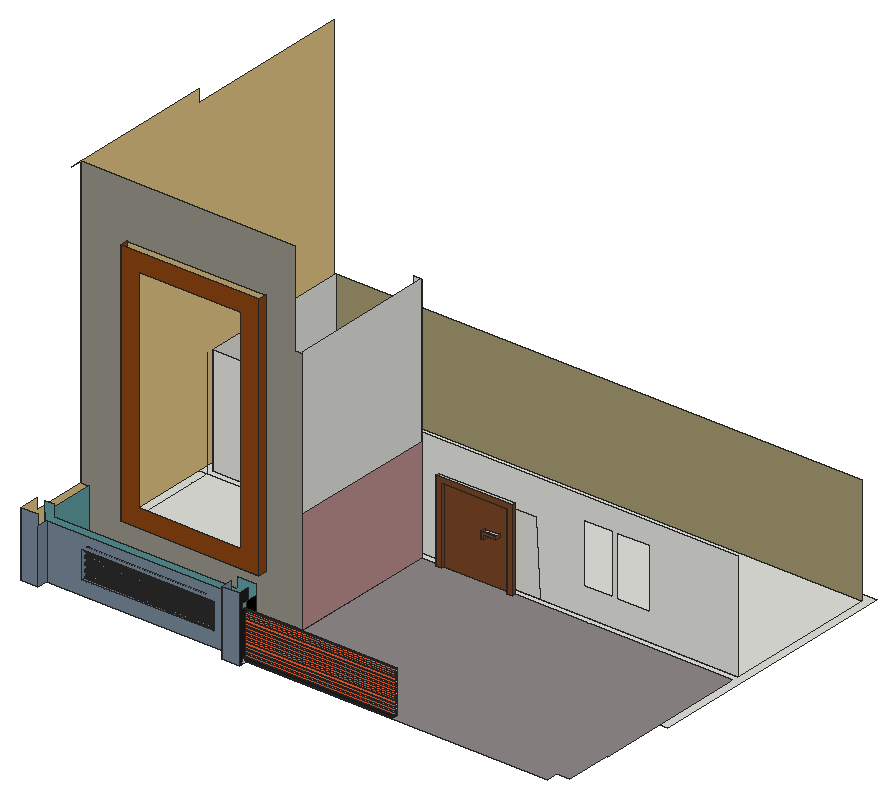
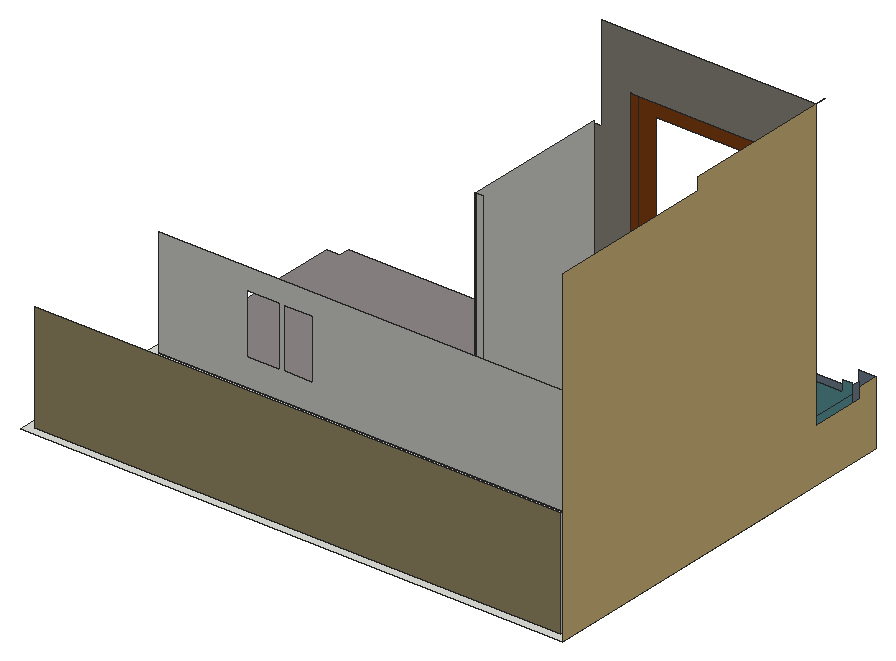
# SketchUp Ruby script. Lengths in inches.
U = 1.inch
M = Sketchup.active_model
def pt(a) = Geom::Point3d.new(a.map { |v| v * U })
def face(e, loops, mat)
  f = e.add_face(loops[0].map { |a| pt(a) })
  loops[1..].each { |l| e.add_face(l.map { |a| pt(a) }).erase! }
  f.material = f.back_material = mat if mat
  f
end
# faces: each face lists its corners as indices into pts; further lists are holes
def faces(e, pts, list, mat = nil) = list.each { |f| face(e, (f[0].is_a?(Array) ? f : [f]).map { |l| l.map { |i| pts[i] } }, mat) }
# xy, xz, yz: faces in a plane at the given z, y or x. An outline is a flat list of corners, or four numbers for a rectangle; further outlines are holes
def ring(l) = l.size == 4 ? [[l[0], l[1]], [l[2], l[1]], [l[2], l[3]], [l[0], l[3]]] : l.each_slice(2).to_a
def flat(e, list, mat, &to3) = list.each { |f| face(e, (f[0].is_a?(Array) ? f : [f]).map { |l| ring(l).map { |u, v| to3.(u, v) } }, mat) }
def xy(e, z, list, mat = nil) = flat(e, list, mat) { |x, y| [x, y, z] }
def xz(e, y, list, mat = nil) = flat(e, list, mat) { |x, z| [x, y, z] }
def yz(e, x, list, mat = nil) = flat(e, list, mat) { |y, z| [x, y, z] }
def lines(e, pts, list) = list.each { |a, b| e.add_line(pt(pts[a]), pt(pts[b])) }
# prism: a flat outline (further loops are holes) pulled along v
def prism(e, loops, v, mat = nil)
  f = face(e, loops, mat); d = Geom::Vector3d.new(v.map { |x| x * U })
  f.pushpull(f.normal.samedirection?(d) ? d.length : -d.length)
end
def box(e, o, s, mat = nil) = prism(e, [[o, [o[0] + s[0], o[1], o[2]], [o[0] + s[0], o[1] + s[1], o[2]], [o[0], o[1] + s[1], o[2]]]], [0, 0, s[2]], mat)
def at(x, y, z, deg = 0) = Geom::Transformation.translation(pt([x, y, z])) * Geom::Transformation.rotation(ORIGIN, Z_AXIS, deg.degrees)
def axes(o, x, y, z) = Geom::Transformation.new([*x, 0, *y, 0, *z, 0, *pt(o).to_a, 1])
def part(name) = M.definitions.add(name)
# library, detail: a bought-in or finely detailed component or shape, given as its bounding box
def library(name, o, s) = part(name).tap { |d| box(d.entities, o, s) }
def detail(e, o, s) = box(e.add_group.entities, o, s)
def put(e, d, t, mat = nil) = e.add_instance(d, t).tap { |i| i.material = mat if mat }
def group(e, t, mat = nil) = e.add_group.tap { |g| g.transformation = t; g.material = mat if mat }.entities
root = M.entities
M.materials.add("[0043_SaddleBrown]").color = [139, 69, 19]
M.materials.add("[0081_CadetBlue]").color = [95, 158, 160]
M.materials.add("[0110_LightSlateGray]").color = [119, 136, 153]
M.materials.add("[0119_RosyBrown]").color = [188, 143, 143]
M.materials.add("[0137_Black]").color = [0, 0, 0]
M.materials.add("[Color B04]").color = [255, 101, 50]
M.materials.add("[Color M08]").color = [30, 30, 30]
M.materials.add("[Concrete Aggregate Smoke]").color = [154, 150, 148]
M.materials.add("[Formica Graystone]").color = [149, 146, 135]
M.materials.add("[Stone Brushed Khaki]").color = [226, 197, 133]
M.materials.add("[Stone Marble]").color = [143, 138, 136]
M.materials.add("[Wood Lumber ButtJoined]").color = [164, 152, 112]
M.materials.add("[Wood Veneer 01]").color = [120, 70, 37]
xy(root,-0.6875,[[249.488,83.423,257.613,247.17]])
xy(root,0,[[12,0,12,83.423,21.531,83.423,21.531,22.384,254.581,22.384,254.581,0,235.107,0,235.107,12,31.287,12,31.287,0],[12,83.423,21,135.461],[21,83.423,249.488,135.461],[249.488,83.423,257.613,135.461],[257.613,83.423,258.19,135.461],
  [12,135.461,21,145.845],[21,135.461,249.488,145.845],[249.488,135.461,257.613,145.845],[257.613,135.461,258.19,145.845],[12,145.845,21,247.17],
  [[603,145.845,603,247.17,355.224,247.17,355.224,250.17,283.224,250.17,283.224,247.17,12,247.17,12,434.423,612,434.423,612,145.845],[21,254.423,603,425.423]],[21,145.845,249.488,247.17],[249.488,145.845,257.613,247.17],[257.613,145.845,258.19,247.17],[276.992,244.17,283.224,247.17],
  [355.224,244.17,361.455,247.17],[283.224,247.17,355.224,250.17],[21,254.423,603,425.423]])
xy(root,0,[[254.581,9.884,587.783,9.884,587.783,22.384,602.489,22.384,602.489,74.423,603,74.423,603,247.17,361.455,247.17,361.455,244.17,355.224,244.17,355.224,247.17,283.224,247.17,283.224,244.17,276.992,244.17,276.992,247.17,258.19,247.17,258.19,83.423,21.531,83.423,21.531,22.384,254.581,22.384]],"[Stone Marble]")
xy(root,4.99,[[254.581,3.884,421.182,9.884]],"[Color M08]")
xy(root,6.884,[[254.581,6.884,420.872,9.884]],"[Color B04]")
xy(root,8.996,[[254.581,6.884,420.872,9.884]],"[Color B04]")
xy(root,10.576,[[254.581,6.884,421.182,9.884]],"[Color B04]")
xy(root,12.688,[[254.581,6.884,421.182,9.884]],"[Color B04]")
xy(root,14.451,[[254.581,6.884,421.182,9.884]],"[Color B04]")
xy(root,15.741,[[70.247,15.6,216.31,19.453],[216.31,15.6,221.935,19.453],[70.247,19.453,216.31,22.384]])
xy(root,15.741,[[70.247,12,216.31,15.6]],"[0110_LightSlateGray]")
xy(root,16.563,[[254.581,6.884,421.182,9.884]],"[Color B04]")
xy(root,18.263,[[254.581,6.884,421.182,9.884]],"[Color B04]")
xy(root,20.375,[[254.581,6.884,421.182,9.884]],"[Color B04]")
xy(root,22.076,[[254.581,6.884,421.182,9.884]],"[Color B04]")
xy(root,24.188,[[254.581,6.884,421.182,9.884]],"[Color B04]")
xy(root,25.888,[[254.581,6.884,421.182,9.884]],"[Color B04]")
xy(root,28,[[254.581,6.884,421.182,9.884]],"[Color B04]")
xy(root,29.701,[[254.581,6.884,421.182,9.884]],"[Color B04]")
xy(root,31.813,[[254.581,6.884,421.182,9.884]],"[Color B04]")
xy(root,33.513,[[254.581,6.884,421.182,9.884]],"[Color B04]")
xy(root,35.625,[[254.581,6.884,421.182,9.884]],"[Color B04]")
xy(root,37.326,[[254.581,6.884,421.182,9.884]],"[Color B04]")
xy(root,39.438,[[254.581,6.884,421.182,9.884]],"[Color B04]")
xy(root,41.138,[[254.581,6.884,421.182,9.884]],"[Color B04]")
xy(root,43.25,[[254.581,6.884,421.182,9.884]],"[Color B04]")
xy(root,43.565,[[63.349,74.423,216.911,83.423]])
xy(root,44.951,[[254.581,6.884,421.182,9.884]],"[Color B04]")
xy(root,45.804,[[70.247,12,216.31,22.384]],"[0110_LightSlateGray]")
xy(root,46.461,[[328.975,241.17,331.645,247.17]],"[Wood Veneer 01]")
xy(root,47.063,[[254.581,6.884,421.182,9.884]],"[Color B04]")
xy(root,48.763,[[254.581,6.884,421.182,9.884]],"[Color B04]")
xy(root,50.875,[[254.581,6.884,421.182,9.884]],"[Color B04]")
xy(root,50.899,[[331.645,241.17,345.538,247.17]],"[Wood Veneer 01]")
xz(root,0,[[12,0,31.287,0,31.287,60,31.228,60,31.228,72,12,72],[235.107,0,254.581,72]],"[0110_LightSlateGray]")
xz(root,6.884,[[254.581,6.884,420.872,8.996],[254.581,10.576,421.182,12.688],[254.581,14.451,421.182,16.563],[254.581,18.263,421.182,20.375],[254.581,22.076,421.182,24.188],
  [254.581,25.888,421.182,28],[254.581,29.701,421.182,31.813],[254.581,33.513,421.182,35.625],[254.581,37.326,421.182,39.438],[254.581,41.138,421.182,43.25],
  [254.581,44.951,421.182,47.063],[254.581,48.763,421.182,50.875]],"[Color B04]")
xz(root,9.884,[[251.209,6.884,254.581,8.996],[254.581,6.884,417.81,8.996],[254.581,10.576,421.182,12.688],[254.581,14.451,421.182,16.563],[254.581,18.263,421.182,20.375],
  [254.581,22.076,421.182,24.188],[254.581,25.888,421.182,28],[254.581,29.701,421.182,31.813],[254.581,33.513,421.182,35.625],[254.581,37.326,421.182,39.438],
  [254.581,41.138,421.182,43.25],[254.581,44.951,421.182,47.063],[254.581,48.763,421.182,50.875]])
xz(root,9.884,[[254.581,4.99,421.182,4.99,421.182,10.576,254.581,10.576,254.581,8.996,420.872,8.996,420.872,6.884,254.581,6.884],[254.581,12.688,421.182,14.451],[254.581,16.563,421.182,18.263],[254.581,20.375,421.182,22.076],[254.581,24.188,421.182,25.888],
  [254.581,28,421.182,29.701],[254.581,31.813,421.182,33.513],[254.581,35.625,421.182,37.326],[254.581,39.438,421.182,41.138],[254.581,43.25,421.182,44.951],
  [254.581,47.063,421.182,48.763],[254.581,50.875,421.182,52.576]],"[Color B04]")
xz(root,12,[[[31.287,0,235.107,60],[70.247,15.741,216.31,45.804]]],"[0110_LightSlateGray]")
xz(root,22.384,[[[21.531,0,21.531,72,31.228,72,31.228,60,235.107,60,235.107,72,254.584,72,254.584,60,254.581,60,254.581,0],[70.247,15.741,216.31,45.804]]],"[0081_CadetBlue]")
xz(root,74.423,[[[63.349,43.565,216.911,317.69],[83.364,63.579,196.897,297.675]]],"[0043_SaddleBrown]")
xz(root,83.423,[[249.488,-0.6875,257.613,0],[21,0,21.531,60],[257.613,0,258.19,273.75]])
xz(root,83.423,[[[21.531,0,257.613,0,257.613,273.75,249.488,273.75,249.488,378.517,12,378.517,12,60,21.531,60],[63.349,43.565,216.911,317.69]]],"[Formica Graystone]")
xz(root,241.17,[[328.975,46.461,331.645,46.461,331.645,50.899,345.538,50.899,345.538,53.899,328.975,53.899]],"[Wood Veneer 01]")
xz(root,244.17,[[276.992,0,283.224,0,283.224,84,355.224,84,355.224,0,361.455,0,361.455,90.231,276.992,90.231]],"[Wood Veneer 01]")
xz(root,247.17,[[249.488,-0.6875,257.613,0],[249.488,0,257.613,276],[257.613,0,258.19,276],[276.992,0,276.992,90.231,361.455,90.231,361.455,0,355.224,0,355.224,84,283.224,84,283.224,0],[328.975,46.461,328.975,53.899,345.538,53.899,345.538,50.899,331.645,50.899,331.645,46.461]])
xz(root,247.17,[[[283.224,0,355.224,84],[328.975,46.461,328.975,53.899,345.538,53.899,345.538,50.899,331.645,50.899,331.645,46.461]]],"[Wood Veneer 01]")
xz(root,250.17,[[283.224,0,355.224,84]])
xz(root,254.423,[[[21,0,603,120],[468.879,30.198,505.379,95.948],[432.379,30.198,464.497,95.948]]])
xz(root,425.423,[[21,0,603,120]],"[Wood Lumber ButtJoined]")
yz(root,12,[[0,0,0,72,22.384,72,22.384,60,83.423,60,83.423,378.517,71.423,378.517,71.423,378.735,247.17,378.735,247.17,364.4375,434.423,364.4375,434.423,0]],"[Stone Brushed Khaki]")
yz(root,21,[[254.423,0,425.423,120]])
yz(root,21.531,[[22.384,0,83.423,60]],"[0081_CadetBlue]")
yz(root,31.287,[[0,0,12,60]],"[0110_LightSlateGray]")
yz(root,63.349,[[74.423,43.565,83.423,317.69]],"[0043_SaddleBrown]")
yz(root,70.247,[[17.526,14.371,18.06,14.441,18.558,14.647,18.985,14.975,19.3125,15.402,19.453,15.741,15.6,15.741,15.74,15.402,16.068,14.975,16.495,14.647,16.992,14.441]])
yz(root,70.247,[[[12,15.741,15.6,15.741,15.534,15.899,15.464,16.433,15.534,16.967,15.74,17.465,16.068,17.892,16.495,18.219,16.992,18.425,17.526,18.496,18.06,18.425,18.558,18.219,18.985,17.892,19.3125,17.465,19.518,16.967,19.589,16.433,19.518,15.899,19.453,15.741,22.384,15.741,22.384,45.804,12,45.804],[17.526,41.121,16.992,41.191,16.495,41.397,16.068,41.725,15.74,42.152,15.534,42.649,15.464,43.183,15.534,43.717,15.74,44.215,16.068,44.642,16.495,44.969,16.992,45.175,17.526,45.246,18.06,45.175,18.558,44.969,18.985,44.642,19.3125,44.215,19.518,43.717,19.589,43.183,19.518,42.649,19.3125,42.152,18.985,41.725,18.558,41.397,18.06,41.191],[17.526,34.433,16.992,34.504,16.495,34.71,16.068,35.037,15.74,35.465,15.534,35.962,15.464,36.496,15.534,37.03,15.74,37.527,16.068,37.954,16.495,38.282,16.992,38.488,17.526,38.558,18.06,38.488,18.558,38.282,18.985,37.954,19.3125,37.527,19.518,37.03,19.589,36.496,19.518,35.962,19.3125,35.465,18.985,35.037,18.558,34.71,18.06,34.504],[17.526,27.746,16.992,27.816,16.495,28.022,16.068,28.35,15.74,28.777,15.534,29.274,15.464,29.808,15.534,30.342,15.74,30.84,16.068,31.267,16.495,31.594,16.992,31.8,17.526,31.871,18.06,31.8,18.558,31.594,18.985,31.267,19.3125,30.84,19.518,30.342,19.589,29.808,19.518,29.274,19.3125,28.777,18.985,28.35,18.558,28.022,18.06,27.816],[17.526,21.058,16.992,21.129,16.495,21.335,16.068,21.662,15.74,22.09,15.534,22.587,15.464,23.121,15.534,23.655,15.74,24.152,16.068,24.579,16.495,24.907,16.992,25.113,17.526,25.183,18.06,25.113,18.558,24.907,18.985,24.579,19.3125,24.152,19.518,23.655,19.589,23.121,19.518,22.587,19.3125,22.09,18.985,21.662,18.558,21.335,18.06,21.129]]],"[0110_LightSlateGray]")
yz(root,216.31,[[[12,15.741,22.384,45.804],[17.526,27.746,18.06,27.816,18.558,28.022,18.985,28.35,19.3125,28.777,19.518,29.274,19.589,29.808,19.518,30.342,19.3125,30.84,18.985,31.267,18.558,31.594,18.06,31.8,17.526,31.871,16.992,31.8,16.495,31.594,16.068,31.267,15.74,30.84,15.534,30.342,15.464,29.808,15.534,29.274,15.74,28.777,16.068,28.35,16.495,28.022,16.992,27.816]]],"[0110_LightSlateGray]")
yz(root,216.911,[[74.423,43.565,83.423,317.69]],"[0043_SaddleBrown]")
yz(root,218.997,[[17.526,21.058,18.06,21.129,18.558,21.335,18.985,21.662,19.3125,22.09,19.518,22.587,19.589,23.121,19.518,23.655,19.3125,24.152,18.985,24.579,18.558,24.907,18.06,25.113,17.526,25.183,16.992,25.113,16.495,24.907,16.068,24.579,15.74,24.152,15.534,23.655,15.464,23.121,15.534,22.587,15.74,22.09,16.068,21.662,16.495,21.335,16.992,21.129]])
yz(root,220.497,[[17.526,41.121,18.06,41.191,18.558,41.397,18.985,41.725,19.3125,42.152,19.518,42.649,19.589,43.183,19.518,43.717,19.3125,44.215,18.985,44.642,18.558,44.969,18.06,45.175,17.526,45.246,16.992,45.175,16.495,44.969,16.068,44.642,15.74,44.215,15.534,43.717,15.464,43.183,15.534,42.649,15.74,42.152,16.068,41.725,16.495,41.397,16.992,41.191]])
yz(root,221.935,[[15.6,15.741,19.453,15.741,19.518,15.899,19.589,16.433,19.518,16.967,19.3125,17.465,18.985,17.892,18.558,18.219,18.06,18.425,17.526,18.496,16.992,18.425,16.495,18.219,16.068,17.892,15.74,17.465,15.534,16.967,15.464,16.433,15.534,15.899]])
yz(root,223.872,[[17.526,34.433,18.06,34.504,18.558,34.71,18.985,35.037,19.3125,35.465,19.518,35.962,19.589,36.496,19.518,37.03,19.3125,37.527,18.985,37.954,18.558,38.282,18.06,38.488,17.526,38.558,16.992,38.488,16.495,38.282,16.068,37.954,15.74,37.527,15.534,37.03,15.464,36.496,15.534,35.962,15.74,35.465,16.068,35.037,16.495,34.71,16.992,34.504]])
yz(root,235.107,[[0,0,12,72]],"[0110_LightSlateGray]")
yz(root,249.488,[[83.423,-0.6875,247.17,0]])
yz(root,254.581,[[3.884,0,6.884,4.99],[6.884,0,9.884,4.99],[6.884,6.884,9.884,8.996],[6.884,10.576,9.884,12.688],[6.884,14.451,9.884,16.563],
  [6.884,18.263,9.884,20.375],[6.884,22.076,9.884,24.188],[6.884,25.888,9.884,28],[6.884,29.701,9.884,31.813],[6.884,33.513,9.884,35.625],
  [6.884,37.326,9.884,39.438],[6.884,41.138,9.884,43.25],[6.884,44.951,9.884,47.063],[6.884,48.763,9.884,50.875]])
yz(root,254.581,[[9.884,0,22.384,60]],"[0137_Black]")
yz(root,254.581,[[0,0,3.884,0,3.884,4.99,9.884,4.99,9.884,6.884,6.884,6.884,6.884,8.996,9.884,8.996,9.884,10.576,6.884,10.576,6.884,12.688,9.884,12.688,9.884,14.451,6.884,14.451,6.884,16.563,9.884,16.563,9.884,18.263,6.884,18.263,6.884,20.375,9.884,20.375,9.884,22.076,6.884,22.076,6.884,24.188,9.884,24.188,9.884,25.888,6.884,25.888,6.884,28,9.884,28,9.884,29.701,6.884,29.701,6.884,31.813,9.884,31.813,9.884,33.513,6.884,33.513,6.884,35.625,9.884,35.625,9.884,37.326,6.884,37.326,6.884,39.438,9.884,39.438,9.884,41.138,6.884,41.138,6.884,43.25,9.884,43.25,9.884,44.951,6.884,44.951,6.884,47.063,9.884,47.063,9.884,48.763,6.884,48.763,6.884,50.875,9.884,50.875,9.884,52.576,6.884,52.576,6.884,54.688,3.884,54.688,3.884,60,12,60,12,72,0,72]],"[Color M08]")
yz(root,257.613,[[83.423,-0.6875,247.17,0],[83.423,0,247.17,276]])
yz(root,258.19,[[83.423,0,247.17,115.0625]],"[0119_RosyBrown]")
yz(root,276.992,[[244.17,0,247.17,90.231]])
yz(root,283.224,[[247.17,0,250.17,84]])
yz(root,283.224,[[244.17,0,247.17,84]],"[Wood Veneer 01]")
yz(root,328.975,[[241.17,46.461,247.17,53.899]],"[Wood Veneer 01]")
yz(root,331.645,[[241.17,46.461,247.17,50.899]],"[Wood Veneer 01]")
yz(root,345.538,[[241.17,50.899,247.17,53.899]],"[Wood Veneer 01]")
yz(root,355.224,[[247.17,0,250.17,84]])
yz(root,355.224,[[244.17,0,247.17,84]],"[Wood Veneer 01]")
yz(root,361.455,[[244.17,0,247.17,90.231]],"[Wood Veneer 01]")
p = [[312,254.423,0],[312,248.307,83.777],[384,248.307,83.777],[384,254.423,0],[70.247,15.534,15.899],[70.247,15.6,15.741],
  [216.31,15.6,15.741],[221.935,15.6,15.741],[221.935,15.534,15.899],[70.247,19.453,15.741],[70.247,19.518,15.899],[221.935,19.518,15.899],
  [221.935,19.453,15.741],[216.31,19.453,15.741],[70.247,15.464,16.433],[221.935,15.464,16.433],[70.247,19.589,16.433],[221.935,19.589,16.433],
  [70.247,15.534,16.967],[221.935,15.534,16.967],[70.247,19.518,16.967],[221.935,19.518,16.967],[70.247,15.74,17.465],[221.935,15.74,17.465],
  [70.247,19.3125,17.465],[221.935,19.3125,17.465],[70.247,16.068,17.892],[221.935,16.068,17.892],[70.247,18.985,17.892],[221.935,18.985,17.892],
  [70.247,16.495,18.219],[221.935,16.495,18.219],[70.247,18.558,18.219],[221.935,18.558,18.219],[70.247,16.992,18.425],[221.935,16.992,18.425],
  [70.247,18.06,18.425],[221.935,18.06,18.425],[70.247,17.526,18.496],[221.935,17.526,18.496],[70.247,16.495,21.335],[70.247,16.992,21.129],
  [218.997,16.992,21.129],[218.997,16.495,21.335],[70.247,17.526,21.058],[218.997,17.526,21.058],[70.247,18.06,21.129],[218.997,18.06,21.129],
  [70.247,18.558,21.335],[218.997,18.558,21.335],[70.247,16.068,21.662],[218.997,16.068,21.662],[70.247,18.985,21.662],[218.997,18.985,21.662],
  [70.247,15.74,22.09],[218.997,15.74,22.09],[70.247,19.3125,22.09],[218.997,19.3125,22.09],[70.247,15.534,22.587],[218.997,15.534,22.587],
  [70.247,19.518,22.587],[218.997,19.518,22.587],[70.247,15.464,23.121],[218.997,15.464,23.121],[70.247,19.589,23.121],[218.997,19.589,23.121],
  [70.247,15.534,23.655],[218.997,15.534,23.655],[70.247,19.518,23.655],[218.997,19.518,23.655],[70.247,15.74,24.152],[218.997,15.74,24.152],
  [70.247,19.3125,24.152],[218.997,19.3125,24.152],[70.247,16.068,24.579],[218.997,16.068,24.579],[70.247,18.985,24.579],[218.997,18.985,24.579],
  [70.247,16.495,24.907],[218.997,16.495,24.907],[70.247,18.558,24.907],[218.997,18.558,24.907],[70.247,16.992,25.113],[218.997,16.992,25.113],
  [70.247,18.06,25.113],[218.997,18.06,25.113],[70.247,17.526,25.183],[218.997,17.526,25.183],[70.247,16.992,27.816],[70.247,17.526,27.746],
  [216.31,17.526,27.746],[216.31,16.992,27.816],[70.247,18.06,27.816],[216.31,18.06,27.816],[70.247,16.495,28.022],[216.31,16.495,28.022],
  [70.247,18.558,28.022],[216.31,18.558,28.022],[70.247,16.068,28.35],[216.31,16.068,28.35],[70.247,18.985,28.35],[216.31,18.985,28.35],
  [70.247,15.74,28.777],[216.31,15.74,28.777],[70.247,19.3125,28.777],[216.31,19.3125,28.777],[70.247,15.534,29.274],[216.31,15.534,29.274],
  [70.247,19.518,29.274],[216.31,19.518,29.274],[70.247,15.464,29.808],[216.31,15.464,29.808],[70.247,19.589,29.808],[216.31,19.589,29.808],
  [70.247,15.534,30.342],[216.31,15.534,30.342],[70.247,19.518,30.342],[216.31,19.518,30.342],[70.247,15.74,30.84],[216.31,15.74,30.84],
  [70.247,19.3125,30.84],[216.31,19.3125,30.84],[70.247,16.068,31.267],[216.31,16.068,31.267],[70.247,18.985,31.267],[216.31,18.985,31.267],
  [70.247,16.495,31.594],[216.31,16.495,31.594],[70.247,18.558,31.594],[216.31,18.558,31.594],[70.247,16.992,31.8],[216.31,16.992,31.8],
  [70.247,18.06,31.8],[216.31,18.06,31.8],[70.247,17.526,31.871],[216.31,17.526,31.871],[70.247,16.992,34.504],[70.247,17.526,34.433],
  [223.872,17.526,34.433],[223.872,16.992,34.504],[70.247,18.06,34.504],[223.872,18.06,34.504],[70.247,16.495,34.71],[223.872,16.495,34.71],
  [70.247,18.558,34.71],[223.872,18.558,34.71],[70.247,16.068,35.037],[223.872,16.068,35.037],[70.247,18.985,35.037],[223.872,18.985,35.037],
  [70.247,15.74,35.465],[223.872,15.74,35.465],[70.247,19.3125,35.465],[223.872,19.3125,35.465],[70.247,15.534,35.962],[223.872,15.534,35.962],
  [70.247,19.518,35.962],[223.872,19.518,35.962],[70.247,15.464,36.496],[223.872,15.464,36.496],[70.247,19.589,36.496],[223.872,19.589,36.496],
  [70.247,15.534,37.03],[223.872,15.534,37.03],[70.247,19.518,37.03],[223.872,19.518,37.03],[70.247,15.74,37.527],[223.872,15.74,37.527],
  [70.247,19.3125,37.527],[223.872,19.3125,37.527],[70.247,16.068,37.954],[223.872,16.068,37.954],[70.247,18.985,37.954],[223.872,18.985,37.954],
  [70.247,16.495,38.282],[223.872,16.495,38.282],[70.247,18.558,38.282],[223.872,18.558,38.282],[70.247,16.992,38.488],[223.872,16.992,38.488],
  [70.247,18.06,38.488],[223.872,18.06,38.488],[70.247,17.526,38.558],[223.872,17.526,38.558],[70.247,16.992,41.191],[70.247,17.526,41.121],
  [220.497,17.526,41.121],[220.497,16.992,41.191],[70.247,18.06,41.191],[220.497,18.06,41.191],[70.247,16.495,41.397],[220.497,16.495,41.397],
  [70.247,18.558,41.397],[220.497,18.558,41.397],[70.247,16.068,41.725],[220.497,16.068,41.725],[70.247,18.985,41.725],[220.497,18.985,41.725],
  [70.247,15.74,42.152],[220.497,15.74,42.152],[70.247,19.3125,42.152],[220.497,19.3125,42.152],[70.247,15.534,42.649],[220.497,15.534,42.649],
  [70.247,19.518,42.649],[220.497,19.518,42.649],[70.247,15.464,43.183],[220.497,15.464,43.183],[70.247,19.589,43.183],[220.497,19.589,43.183],
  [70.247,15.534,43.717],[220.497,15.534,43.717],[70.247,19.518,43.717],[220.497,19.518,43.717],[70.247,15.74,44.215],[220.497,15.74,44.215],
  [70.247,19.3125,44.215],[220.497,19.3125,44.215],[70.247,16.068,44.642],[220.497,16.068,44.642],[70.247,18.985,44.642],[220.497,18.985,44.642],
  [70.247,16.495,44.969],[220.497,16.495,44.969],[70.247,18.558,44.969],[220.497,18.558,44.969],[70.247,16.992,45.175],[220.497,16.992,45.175],
  [70.247,18.06,45.175],[220.497,18.06,45.175],[70.247,17.526,45.246],[220.497,17.526,45.246],[21,247.17,120],[21,247.17,0]]
faces(root,p,[[0,1,2,3]])
faces(root,p,[[4,5,6,7,8],[9,10,11,12,13],[14,4,8,15],[10,16,17,11],[18,14,15,19],[16,20,21,17],[22,18,19,23],[20,24,25,21],
  [26,22,23,27],[24,28,29,25],[30,26,27,31],[28,32,33,29],[34,30,31,35],[32,36,37,33],[38,34,35,39],[36,38,39,37],
  [40,41,42,43],[41,44,45,42],[44,46,47,45],[46,48,49,47],[50,40,43,51],[48,52,53,49],[54,50,51,55],[52,56,57,53],
  [58,54,55,59],[56,60,61,57],[62,58,59,63],[60,64,65,61],[66,62,63,67],[64,68,69,65],[70,66,67,71],[68,72,73,69],
  [74,70,71,75],[72,76,77,73],[78,74,75,79],[76,80,81,77],[82,78,79,83],[80,84,85,81],[86,82,83,87],[84,86,87,85],
  [88,89,90,91],[89,92,93,90],[94,88,91,95],[92,96,97,93],[98,94,95,99],[96,100,101,97],[102,98,99,103],[100,104,105,101],
  [106,102,103,107],[104,108,109,105],[110,106,107,111],[108,112,113,109],[114,110,111,115],[112,116,117,113],[118,114,115,119],[116,120,121,117],
  [122,118,119,123],[120,124,125,121],[126,122,123,127],[124,128,129,125],[130,126,127,131],[128,132,133,129],[134,130,131,135],[132,134,135,133],
  [136,137,138,139],[137,140,141,138],[142,136,139,143],[140,144,145,141],[146,142,143,147],[144,148,149,145],[150,146,147,151],[148,152,153,149],
  [154,150,151,155],[152,156,157,153],[158,154,155,159],[156,160,161,157],[162,158,159,163],[160,164,165,161],[166,162,163,167],[164,168,169,165],
  [170,166,167,171],[168,172,173,169],[174,170,171,175],[172,176,177,173],[178,174,175,179],[176,180,181,177],[182,178,179,183],[180,182,183,181],
  [184,185,186,187],[185,188,189,186],[190,184,187,191],[188,192,193,189],[194,190,191,195],[192,196,197,193],[198,194,195,199],[196,200,201,197],
  [202,198,199,203],[200,204,205,201],[206,202,203,207],[204,208,209,205],[210,206,207,211],[208,212,213,209],[214,210,211,215],[212,216,217,213],
  [218,214,215,219],[216,220,221,217],[222,218,219,223],[220,224,225,221],[226,222,223,227],[224,228,229,225],[230,226,227,231],[228,230,231,229]],"[Concrete Aggregate Smoke]")
lines(root,p,[[232,233]])
